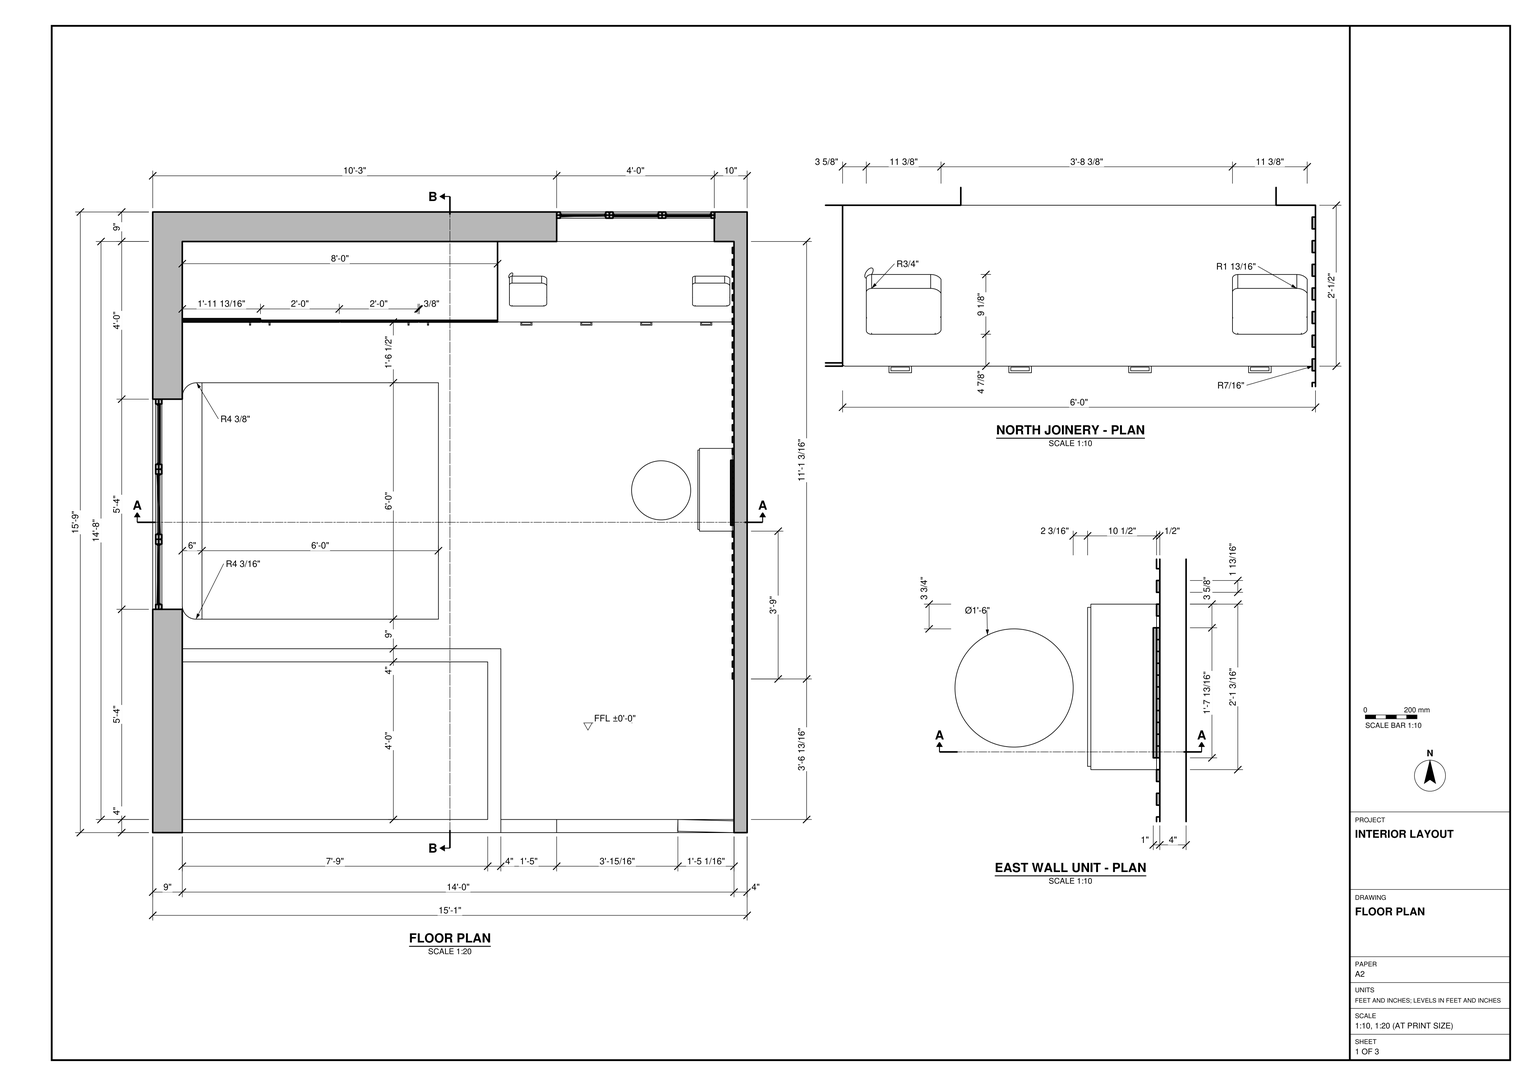
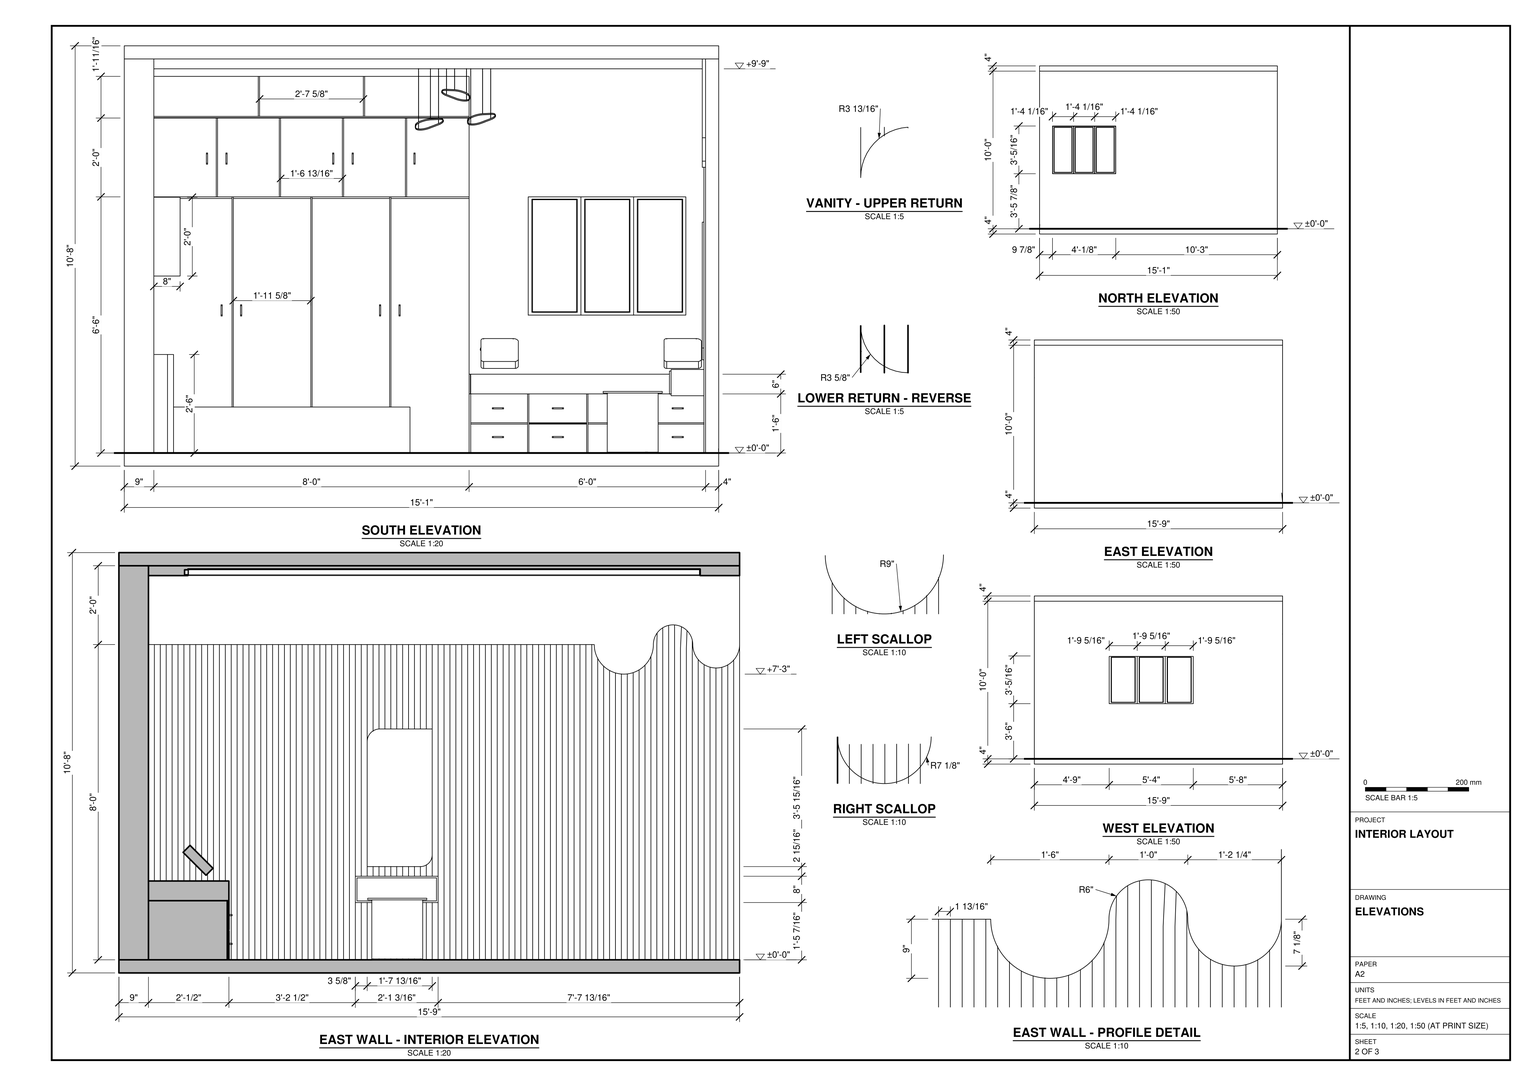
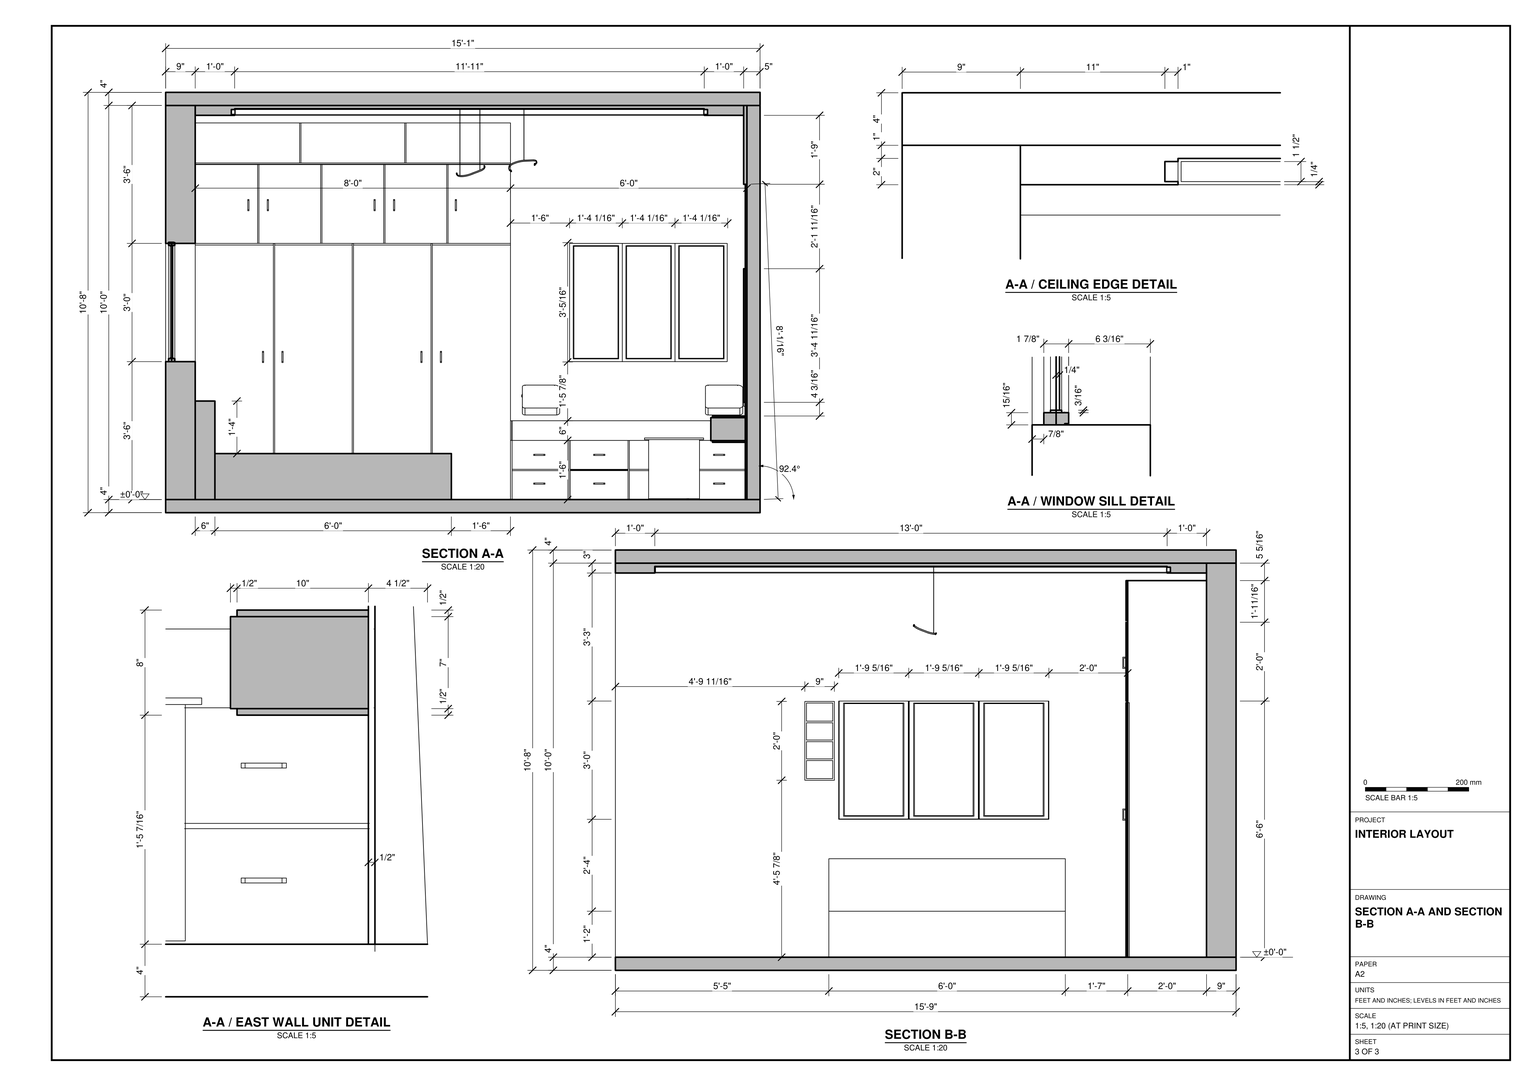
Build the bedroom interior in SketchUp from task_files/diagram_01.pdf. Work in feet and inches. Set the finished floor at ±0'-0". The overall model is 15'-1" east to west, 15'-9" north to south and 10'-8" high. Use the floor plan to locate the walls and furniture, and the elevations and sections to set their heights.

Model the floor slab, the 9" north and west walls, the 4" east wall and the top slab. Keep the south side open as drawn. Include the stepped ceiling edge and the three-panel window units in the north and west walls. Place the platform bed with its headboard against the west wall beneath the window. Along the north wall, fit the tall wardrobe and overhead cupboards beside the low drawer unit, keeping the opening below its counter in the position shown.

On the east wall, model the vertical ribs and follow the profile detail where their upper edge curves. Place the shallow dressing unit and mirror against this wall, with the round stool in front. Include the pendant lights in the position shown in elevation. Decor and loose items, including lights, may be any suitable library components.

Keep shell elements and each furniture or joinery piece in separate groups or components, and use components for repeated parts. Save one SketchUp model as output_files/bedroom_with_fitted_storage_and_a_dressing_area.skp.

# SketchUp Ruby script. Lengths in inches.
U = 1.inch
M = Sketchup.active_model
def pt(a) = Geom::Point3d.new(a.map { |v| v * U })
def face(e, loops, mat)
  f = e.add_face(loops[0].map { |a| pt(a) })
  loops[1..].each { |l| e.add_face(l.map { |a| pt(a) }).erase! }
  f.material = f.back_material = mat if mat
  f
end
# faces: each face lists its corners as indices into pts; further lists are holes
def faces(e, pts, list, mat = nil) = list.each { |f| face(e, (f[0].is_a?(Array) ? f : [f]).map { |l| l.map { |i| pts[i] } }, mat) }
# xy, xz, yz: faces in a plane at the given z, y or x. An outline is a flat list of corners, or four numbers for a rectangle; further outlines are holes
def ring(l) = l.size == 4 ? [[l[0], l[1]], [l[2], l[1]], [l[2], l[3]], [l[0], l[3]]] : l.each_slice(2).to_a
def flat(e, list, mat, &to3) = list.each { |f| face(e, (f[0].is_a?(Array) ? f : [f]).map { |l| ring(l).map { |u, v| to3.(u, v) } }, mat) }
def xy(e, z, list, mat = nil) = flat(e, list, mat) { |x, y| [x, y, z] }
def xz(e, y, list, mat = nil) = flat(e, list, mat) { |x, z| [x, y, z] }
def yz(e, x, list, mat = nil) = flat(e, list, mat) { |y, z| [x, y, z] }
def lines(e, pts, list) = list.each { |a, b| e.add_line(pt(pts[a]), pt(pts[b])) }
# prism: a flat outline (further loops are holes) pulled along v
def prism(e, loops, v, mat = nil)
  f = face(e, loops, mat); d = Geom::Vector3d.new(v.map { |x| x * U })
  f.pushpull(f.normal.samedirection?(d) ? d.length : -d.length)
end
def box(e, o, s, mat = nil) = prism(e, [[o, [o[0] + s[0], o[1], o[2]], [o[0] + s[0], o[1] + s[1], o[2]], [o[0], o[1] + s[1], o[2]]]], [0, 0, s[2]], mat)
def at(x, y, z, deg = 0) = Geom::Transformation.translation(pt([x, y, z])) * Geom::Transformation.rotation(ORIGIN, Z_AXIS, deg.degrees)
def axes(o, x, y, z) = Geom::Transformation.new([*x, 0, *y, 0, *z, 0, *pt(o).to_a, 1])
def part(name) = M.definitions.add(name)
# library, detail: a bought-in or finely detailed component or shape, given as its bounding box
def library(name, o, s) = part(name).tap { |d| box(d.entities, o, s) }
def detail(e, o, s) = box(e.add_group.entities, o, s)
def put(e, d, t, mat = nil) = e.add_instance(d, t).tap { |i| i.material = mat if mat }
def group(e, t, mat = nil) = e.add_group.tap { |g| g.transformation = t; g.material = mat if mat }.entities
root = M.entities
M.materials.add("0130_Gainsboro").color = [39, 45, 50]
M.materials.add("Emissive").color = [240, 235, 85]
M.materials.add("Wine2").color = [0, 0, 0]
M.materials["Wine2"].alpha = 0
M.materials.add("[0055_LightGoldenrodYellow]").color = [250, 250, 210]
M.materials.add("[0066_Honeydew]").color = [240, 255, 240]
M.materials.add("[0067_PaleGreen]").color = [223, 240, 176]
M.materials.add("[0134_DimGray]").color = [105, 105, 105]
M.materials.add("[Aluminum]").color = [179, 179, 179]
M.materials.add("[Carpet Berber Multi]").color = [151, 134, 122]
M.materials.add("[Carpet Berber Pattern Gray]").color = [165, 165, 165]
M.materials.add("[Carpet Pattern Leaf Squares Tan]").color = [181, 154, 125]
M.materials.add("[Carpet Pattern Squares Multi]").color = [138, 129, 101]
M.materials.add("[Mirror 02]").color = [229, 229, 229]
M.materials.add("[Translucent Glass Sky Reflection]").color = [126, 138, 183]
M.materials["[Translucent Glass Sky Reflection]"].alpha = 0.52
c1 = library("Rectangle Light",[-5.15,-5.15,-5.15],[10.3,10.3,5.15])
c2 = library("pendants",[20.82,-32.18,-15.09],[139.89,104.33,117.98])
c3 = part("Wardrobe door panel")
xy(c3.entities,0,[[0,-0.98,43.07,0],[0,0,43.07,1.4]],"0130_Gainsboro")
xy(c3.entities,0.3,[[0.3,-1.43,42.77,-0.98]],"0130_Gainsboro")
xy(c3.entities,2.95,[[2.95,-1.43,40.12,-0.63],[2.95,-0.63,40.12,0],[2.95,0,40.12,0.64],[2.95,0.64,40.12,1.4]],"0130_Gainsboro")
xy(c3.entities,3.54,[[3.54,-0.63,39.53,0],[3.54,0,39.53,0.64]],"0130_Gainsboro")
xy(c3.entities,111.8125,[[3.54,-0.63,39.53,0],[3.54,0,39.53,0.64]],"0130_Gainsboro")
xy(c3.entities,112.4,[[2.95,-1.43,40.12,-0.63],[2.95,-0.63,40.12,0],[2.95,0,40.12,0.64],[2.95,0.64,40.12,1.4]],"0130_Gainsboro")
xy(c3.entities,115.05,[[0.3,-1.43,42.77,-0.98]],"0130_Gainsboro")
xy(c3.entities,115.35,[[0,-0.98,43.07,0],[0,0,43.07,1.4]],"0130_Gainsboro")
xz(c3.entities,-1.43,[[[0.3,0.3,42.77,115.05],[2.95,2.95,40.12,112.4]]],"0130_Gainsboro")
xz(c3.entities,-0.98,[[[0,0,43.07,115.35],[0.3,0.3,42.77,115.05]]],"0130_Gainsboro")
xz(c3.entities,-0.63,[[[2.95,2.95,40.12,112.4],[3.54,3.54,39.53,111.8125]]],"0130_Gainsboro")
xz(c3.entities,0,[[[0,0,43.07,115.35],[2.95,2.95,40.12,112.4]],[[2.95,2.95,40.12,112.4],[3.54,3.54,39.53,111.8125]]],"0130_Gainsboro")
xz(c3.entities,0,[[3.54,3.54,39.53,111.8125]],"Wine2")
xz(c3.entities,0.64,[[[2.95,2.95,40.12,112.4],[3.54,3.54,39.53,111.8125]]],"0130_Gainsboro")
xz(c3.entities,1.4,[[[0,0,43.07,115.35],[2.95,2.95,40.12,112.4]]],"0130_Gainsboro")
yz(c3.entities,0,[[-0.98,0,0,115.35],[0,0,1.4,115.35]],"0130_Gainsboro")
yz(c3.entities,0.3,[[-1.43,0.3,-0.98,115.05]],"0130_Gainsboro")
yz(c3.entities,2.95,[[-1.43,2.95,-0.63,112.4],[-0.63,2.95,0,112.4],[0,2.95,0.64,112.4],[0.64,2.95,1.4,112.4]],"0130_Gainsboro")
yz(c3.entities,3.54,[[-0.63,3.54,0,111.8125],[0,3.54,0.64,111.8125]],"0130_Gainsboro")
yz(c3.entities,39.53,[[-0.63,3.54,0,111.8125],[0,3.54,0.64,111.8125]],"0130_Gainsboro")
yz(c3.entities,40.12,[[-1.43,2.95,-0.63,112.4],[-0.63,2.95,0,112.4],[0,2.95,0.64,112.4],[0.64,2.95,1.4,112.4]],"0130_Gainsboro")
yz(c3.entities,42.77,[[-1.43,0.3,-0.98,115.05]],"0130_Gainsboro")
yz(c3.entities,43.07,[[-0.98,0,0,115.35],[0,0,1.4,115.35]],"0130_Gainsboro")
c4 = part("Wardrobe door assembly")
put(c4.entities,c3,axes([90.57,1.43,0],[1.05148,0,0],[0,1,0],[0,0,1]))
put(c4.entities,c3,axes([0,1.43,0],[1.05148,0,0],[0,1,0],[0,0,1]))
put(c4.entities,c3,axes([45.29,1.43,0],[1.05148,0,0],[0,1,0],[0,0,1]))
c5 = part("Group\#8")
prism(c5.entities,[[[0,1,3.4375],[0,1,0],[0,0,0],[0,0,3.4375]],[[0,0.86,3.14],[0,0.29,3.14],[0,0.29,0.33],[0,0.86,0.33]]],[0.375,0,0])
c6 = library("Group\#13",[0,0,0],[1,180,33])
c7 = library("Group\#17",[0,0,0],[15.5,15.5,18])
c8 = library("Group\#18",[0,0,0],[18,18,0.5])
xy(root,4,[[123,0,159.92,0,159.92,0.41,159.83,0.41,159.92,4,123,4],[177,0,177.09,3.59,159.92,4,159.92,0.41],[159.83,0.41,159.92,0.41,159.92,4],[9,155.5,32.8,156.5],[33.2,155.5,56.8,156],
  [57.2,155.5,80.8,156]])
xy(root,81.5,[[9,155.5,32.8,156.5],[33.2,155.5,56.8,156],[57.2,155.5,80.8,156]])
xz(root,156,[[33.2,4,56.8,81.5],[57.2,4,80.8,81.5]])
xz(root,156.5,[[9,4,32.8,81.5]])
xz(root,187.62,[[140.37,47.02,153.78,81.125],[156.42,47.02,169.83,81.125]],"[Translucent Glass Sky Reflection]")
yz(root,2.25,[[112.42,47.12,130.25,81.22]],"[Translucent Glass Sky Reflection]")
yz(root,9,[[155.5,4,156.5,81.5]])
yz(root,32.8,[[155.5,4,156.5,81.5]])
yz(root,33.2,[[155.5,4,156,81.5]])
yz(root,56.8,[[155.5,4,156,81.5]])
yz(root,57.2,[[155.5,4,156,81.5]])
yz(root,80.8,[[155.5,4,156,81.5]])
# 1 loose lines left out
p = [[124.32,187.62,81.125],[124.32,187.62,47.02],[137.73,188.05,47.02],[137.73,188.05,81.125],[1.83,87.58,47.12],[1.83,87.58,81.22],
  [1.4,69.75,81.22],[1.4,69.75,47.12],[2.25,91.09,47.11],[1.4,108.91,47.11],[1.4,108.91,81.22],[2.25,91.09,81.22]]
faces(root,p,[[0,1,2,3],[4,5,6,7],[8,9,10,11]],"[Translucent Glass Sky Reflection]")
put(root,c1,axes([15.1,9.07,120.99],[0.8,0,0],[0,0.8,0],[0,0,0.8]))
put(root,c1,axes([15.1,76.48,120.99],[0.8,0,0],[0,0.8,0],[0,0,0.8]))
put(root,c1,axes([15.1,143.89,120.99],[0.8,0,0],[0,0.8,0],[0,0,0.8]))
put(root,c1,axes([169.6,76.48,120.99],[0.8,0,0],[0,0.8,0],[0,0,0.8]))
put(root,c1,axes([169.6,143.89,120.99],[0.8,0,0],[0,0.8,0],[0,0,0.8]))
put(root,c1,axes([169.6,9.07,120.99],[0.8,0,0],[0,0.8,0],[0,0,0.8]))
put(root,c1,axes([140.91,173.9,121],[0.8,0,0],[0,0.8,0],[0,0,0.8]))
put(root,c2,axes([84.45,87.32,104.48],[0.18,0,0],[0,0.18,0],[0,0,0.18]))
put(root,c4,axes([2.78,68,46],[0,0.47107,0],[-0.6678,0,0],[0,0,0.315]))
put(root,c4,axes([171.15,189,45.9],[-0.35441,0,0],[0,-0.6678,0],[0,0,0.315]))
g1 = group(root,at(9,156,4))
xy(g1,0,[[0,0,96,24]])
xy(g1,114.6875,[[0,0,96,24]])
xz(g1,0,[[0,0,23.8,78],[23.8,0,24.2,78],[24.2,0,47.8,78],[47.8,0,48.2,78],[48.2,0,71.8,78],
  [71.8,0,72.2,78],[72.2,0,96,78],[0,78,96,102.125],[0,102.125,96,114.6875]])
xz(g1,24,[[0,0,96,114.6875]])
yz(g1,0,[[0,0,24,114.6875]])
yz(g1,96,[[0,0,24,114.6875]])
g2 = group(root,at(9,155.5,4),"[0055_LightGoldenrodYellow]")
box(g2,[19.4,0,78],[18.8,0.5,24])
box(g2,[38.6,0,78],[18.8,0.5,24])
box(g2,[57.8,0,78],[18.8,0.5,24])
xy(g2,78,[[0,0,19,0.5]])
xy(g2,102,[[0,0,19,0.5]])
xz(g2,0,[[0,0,23.8,77.5],[24.2,0,47.8,77.5],[48.2,0,71.8,77.5],[72.2,0,96,77.5],[[0,78,19,102],[16,87.9375,16.375,91.375]],
  [77,78,96,102],[16,87.9375,16.375,91.375]])
xz(g2,0.5,[[0,78,19,102]])
yz(g2,0,[[0,78,0.5,102]])
yz(g2,19,[[0,78,0.5,102]])
put(root,c5,at(25,154.5,91.9375),"[Aluminum]")
put(root,c5,at(30.9375,154.5,91.9375),"[Aluminum]")
put(root,c5,at(63.4375,154.5,91.9375),"[Aluminum]")
put(root,c5,at(69.375,154.5,91.9375),"[Aluminum]")
put(root,c5,at(29.46,154.5,45.71),"[Aluminum]")
put(root,c5,at(35.39,154.5,45.71),"[Aluminum]")
put(root,c5,at(77.71,154.5,45.71),"[Aluminum]")
put(root,c5,at(83.64,154.5,45.71),"[Aluminum]")
put(root,c5,at(88.1875,154.5,91.9375))
g3 = group(root,at(9,65,4),"[Carpet Berber Pattern Gray]")
xy(g3,0,[[4.03,0,3.64,0.03,3.38,0.07,3.25,0.1,3.125,0.13,3,0.17,2.875,0.2,2.75,0.25,2.63,0.29,2.51,0.34,2.39,0.4,2.27,0.45,2.16,0.51,2.04,0.58,1.82,0.72,1.72,0.79,1.61,0.875,1.51,0.96,1.41,1.04,1.3125,1.13,1.22,1.22,1.13,1.3125,1.04,1.41,0.96,1.51,0.875,1.61,0.79,1.72,0.72,1.82,0.58,2.04,0.51,2.16,0.45,2.27,0.4,2.39,0.34,2.51,0.29,2.63,0.25,2.75,0.2,2.875,0.17,3,0.13,3.125,0.1,3.25,0.07,3.38,0.03,3.64,0,4.03,0,67.77,0.02,68.05,0.03,68.18,0.05,68.32,0.08,68.45,0.11,68.59,0.17,68.85,0.21,68.98,0.36,69.37,0.42,69.49,0.48,69.62,0.54,69.74,0.61,69.86,0.68,69.97,0.75,70.09,0.83,70.2,0.92,70.31,1,70.42,1.18,70.62,1.38,70.82,1.58,71,1.69,71.08,1.8,71.17,1.91,71.25,2.03,71.32,2.14,71.39,2.26,71.46,2.38,71.52,2.51,71.58,2.63,71.64,3.02,71.79,3.15,71.83,3.41,71.89,3.55,71.92,3.68,71.95,3.82,71.97,3.95,71.98,4.23,72,6,72,6,0],[6,0,78,72]])
xy(g3,14,[[6,0,78,72]])
xy(g3,30,[[4.03,0,6,0,6,72,4.23,72,3.95,71.98,3.82,71.97,3.68,71.95,3.55,71.92,3.41,71.89,3.15,71.83,3.02,71.79,2.63,71.64,2.51,71.58,2.38,71.52,2.26,71.46,2.14,71.39,2.03,71.32,1.91,71.25,1.8,71.17,1.69,71.08,1.58,71,1.38,70.82,1.18,70.62,1,70.42,0.92,70.31,0.83,70.2,0.75,70.09,0.68,69.97,0.61,69.86,0.54,69.74,0.48,69.62,0.42,69.49,0.36,69.37,0.21,68.98,0.17,68.85,0.11,68.59,0.08,68.45,0.05,68.32,0.03,68.18,0.02,68.05,0,67.77,0,4.03,0.03,3.64,0.07,3.38,0.1,3.25,0.13,3.125,0.17,3,0.2,2.875,0.25,2.75,0.29,2.63,0.34,2.51,0.4,2.39,0.45,2.27,0.51,2.16,0.58,2.04,0.72,1.82,0.79,1.72,0.875,1.61,0.96,1.51,1.04,1.41,1.13,1.3125,1.22,1.22,1.3125,1.13,1.41,1.04,1.51,0.96,1.61,0.875,1.72,0.79,1.82,0.72,2.04,0.58,2.16,0.51,2.27,0.45,2.39,0.4,2.51,0.34,2.63,0.29,2.75,0.25,2.875,0.2,3,0.17,3.125,0.13,3.25,0.1,3.38,0.07,3.64,0.03]])
xz(g3,0,[[4.03,0,4.16,30],[4.16,0,6,30],[6,0,78,14]])
xz(g3,72,[[4.23,0,4.37,30],[4.37,0,6,30],[6,0,78,14]])
yz(g3,0,[[4.03,0,4.16,30],[4.16,0,67.63,30],[67.63,0,67.77,30]])
yz(g3,6,[[0,0,72,14],[0,14,72,30]])
yz(g3,78,[[0,0,72,14]])
# 2 loose lines left out
p = [[3.51,0.05,0],[3.64,0.03,0],[3.64,0.03,30],[3.51,0.05,30],[3.77,0.02,0],[3.77,0.02,30],
  [3.9,0.01,0],[3.9,0.01,30],[4.03,0,0],[4.03,0,30],[3,0.17,0],[3.125,0.13,0],
  [3.125,0.13,30],[3,0.17,30],[3.25,0.1,0],[3.25,0.1,30],[3.38,0.07,0],[3.38,0.07,30],
  [2.63,0.29,0],[2.75,0.25,0],[2.75,0.25,30],[2.63,0.29,30],[2.875,0.2,0],[2.875,0.2,30],
  [2.39,0.4,0],[2.51,0.34,0],[2.51,0.34,30],[2.39,0.4,30],[2.27,0.45,0],[2.27,0.45,30],
  [2.04,0.58,0],[2.16,0.51,0],[2.16,0.51,30],[2.04,0.58,30],[1.82,0.72,0],[1.93,0.65,0],
  [1.93,0.65,30],[1.82,0.72,30],[1.72,0.79,0],[1.72,0.79,30],[1.61,0.875,0],[1.61,0.875,30],
  [1.51,0.96,0],[1.51,0.96,30],[1.3125,1.13,0],[1.41,1.04,0],[1.41,1.04,30],[1.3125,1.13,30],
  [1.22,1.22,0],[1.22,1.22,30],[1.13,1.3125,0],[1.13,1.3125,30],[1.04,1.41,0],[1.04,1.41,30],
  [0.96,1.51,0],[0.96,1.51,30],[0.875,1.61,0],[0.875,1.61,30],[0.79,1.72,0],[0.79,1.72,30],
  [0.72,1.82,0],[0.72,1.82,30],[0.65,1.93,0],[0.65,1.93,30],[0.58,2.04,0],[0.58,2.04,30],
  [0.51,2.16,0],[0.51,2.16,30],[0.45,2.27,0],[0.45,2.27,30],[0.4,2.39,0],[0.4,2.39,30],
  [0.34,2.51,0],[0.34,2.51,30],[0.29,2.63,0],[0.29,2.63,30],[0.25,2.75,0],[0.25,2.75,30],
  [0.2,2.875,0],[0.2,2.875,30],[0.17,3,0],[0.17,3,30],[0.13,3.125,0],[0.13,3.125,30],
  [0.1,3.25,0],[0.1,3.25,30],[0.07,3.38,0],[0.07,3.38,30],[0.05,3.51,0],[0.05,3.51,30],
  [0.03,3.64,0],[0.03,3.64,30],[0.02,3.77,0],[0.02,3.77,30],[0.01,3.9,0],[0.01,3.9,30],
  [0,4.03,0],[0,4.03,30],[0.01,67.91,0],[0,67.77,0],[0,67.77,30],[0.01,67.91,30],
  [0.02,68.05,0],[0.02,68.05,30],[0.03,68.18,0],[0.03,68.18,30],[0.05,68.32,0],[0.05,68.32,30],
  [0.08,68.45,0],[0.08,68.45,30],[0.11,68.59,0],[0.11,68.59,30],[0.14,68.72,0],[0.14,68.72,30],
  [0.17,68.85,0],[0.17,68.85,30],[0.21,68.98,0],[0.21,68.98,30],[0.26,69.11,0],[0.26,69.11,30],
  [0.31,69.24,0],[0.31,69.24,30],[0.36,69.37,0],[0.36,69.37,30],[0.42,69.49,0],[0.42,69.49,30],
  [0.48,69.62,0],[0.48,69.62,30],[0.54,69.74,0],[0.54,69.74,30],[0.61,69.86,0],[0.61,69.86,30],
  [0.68,69.97,0],[0.68,69.97,30],[0.75,70.09,0],[0.75,70.09,30],[0.83,70.2,0],[0.83,70.2,30],
  [0.92,70.31,0],[0.92,70.31,30],[1,70.42,0],[1,70.42,30],[1.09,70.52,0],[1.09,70.52,30],
  [1.18,70.62,0],[1.18,70.62,30],[1.28,70.72,0],[1.28,70.72,30],[1.38,70.82,0],[1.38,70.82,30],
  [1.48,70.91,0],[1.48,70.91,30],[1.58,71,0],[1.58,71,30],[1.69,71.08,0],[1.69,71.08,30],
  [1.8,71.17,0],[1.8,71.17,30],[1.91,71.25,0],[1.91,71.25,30],[2.03,71.32,0],[2.03,71.32,30],
  [2.14,71.39,0],[2.14,71.39,30],[2.26,71.46,0],[2.26,71.46,30],[2.38,71.52,0],[2.38,71.52,30],
  [2.51,71.58,0],[2.51,71.58,30],[2.63,71.64,0],[2.63,71.64,30],[2.76,71.69,0],[2.76,71.69,30],
  [2.89,71.74,0],[2.89,71.74,30],[3.02,71.79,0],[3.02,71.79,30],[3.15,71.83,0],[3.15,71.83,30],
  [3.28,71.86,0],[3.28,71.86,30],[3.41,71.89,0],[3.41,71.89,30],[3.55,71.92,0],[3.55,71.92,30],
  [3.68,71.95,0],[3.68,71.95,30],[3.82,71.97,0],[3.82,71.97,30],[3.95,71.98,0],[3.95,71.98,30],
  [4.09,71.99,0],[4.09,71.99,30],[4.23,72,0],[4.23,72,30]]
faces(g3,p,[[0,1,2,3],[1,4,5,2],[4,6,7,5],[6,8,9,7],[10,11,12,13],[11,14,15,12],[14,16,17,15],[16,0,3,17],
  [18,19,20,21],[19,22,23,20],[22,10,13,23],[24,25,26,27],[25,18,21,26],[28,24,27,29],[30,31,32,33],[31,28,29,32],
  [34,35,36,37],[35,30,33,36],[38,34,37,39],[40,38,39,41],[42,40,41,43],[44,45,46,47],[45,42,43,46],[48,44,47,49],
  [50,48,49,51],[52,50,51,53],[54,52,53,55],[56,54,55,57],[58,56,57,59],[60,58,59,61],[62,60,61,63],[64,62,63,65],
  [66,64,65,67],[68,66,67,69],[70,68,69,71],[72,70,71,73],[74,72,73,75],[76,74,75,77],[78,76,77,79],[80,78,79,81],
  [82,80,81,83],[84,82,83,85],[86,84,85,87],[88,86,87,89],[90,88,89,91],[92,90,91,93],[94,92,93,95],[96,94,95,97],
  [98,99,100,101],[102,98,101,103],[104,102,103,105],[106,104,105,107],[108,106,107,109],[110,108,109,111],[112,110,111,113],[114,112,113,115],
  [116,114,115,117],[118,116,117,119],[120,118,119,121],[122,120,121,123],[124,122,123,125],[126,124,125,127],[128,126,127,129],[130,128,129,131],
  [132,130,131,133],[134,132,133,135],[136,134,135,137],[138,136,137,139],[140,138,139,141],[142,140,141,143],[144,142,143,145],[146,144,145,147],
  [148,146,147,149],[150,148,149,151],[152,150,151,153],[154,152,153,155],[156,154,155,157],[158,156,157,159],[160,158,159,161],[162,160,161,163],
  [164,162,163,165],[166,164,165,167],[168,166,167,169],[170,168,169,171],[172,170,171,173],[174,172,173,175],[176,174,175,177],[178,176,177,179],
  [180,178,179,181],[182,180,181,183],[184,182,183,185],[186,184,185,187],[188,186,187,189],[190,188,189,191],[192,190,191,193],[194,192,193,195]])
g4 = group(root,at(81.2,155.5,4))
xy(g4,0,[[0,0,23.8,0.5],[23.8,0.5,95.8,24.5]])
xy(g4,18,[[23.8,0.5,95.8,24.5]])
xy(g4,77.5,[[0,0,23.8,0.5]])
xz(g4,0.5,[[0,0,23.8,77.4],[23.8,0,24.3,18],[24.3,0,41.6,18],[41.6,0,42,18],[42,0,59.6,18],
  [59.6,0,60,18],[60,0,77.6,18],[77.6,0,78,18],[78,0,95.8,18],[0,77.4,23.8,77.5]])
xz(g4,24.5,[[23.8,0,95.8,18]])
yz(g4,0,[[0,0,0.5,77.4],[0,77.4,0.5,77.5]])
yz(g4,23.8,[[0,0,0.5,77.4],[0.5,0,24.5,18],[0,77.4,0.5,77.5]])
yz(g4,95.8,[[0.5,0,24.5,18]])
put(root,c5,axes([115.5,154.5,17.42],[0,0,1],[0,1,0],[-1,0,0]),"[Aluminum]")
put(root,c5,axes([133.75,154.5,17.42],[0,0,1],[0,1,0],[-1,0,0]),"[Aluminum]")
g5 = group(root,at(152,154.5,17.42),"[Aluminum]")
prism(g5,[[[-3.4375,1,0],[0,1,0],[0,0,0],[-3.4375,0,0]],[[-3.14,0.86,0],[-3.14,0.29,0],[-0.33,0.29,0],[-0.33,0.86,0]]],[0,0,0.375])
put(root,c5,axes([170.25,154.5,17.42],[0,0,1],[0,1,0],[-1,0,0]),"[Aluminum]")
put(root,c5,axes([115.5,154.5,8.67],[0,0,1],[0,1,0],[-1,0,0]),"[Aluminum]")
put(root,c5,axes([133.75,154.5,8.67],[0,0,1],[0,1,0],[-1,0,0]),"[Aluminum]")
put(root,c5,axes([170.25,154.5,8.67],[0,0,1],[0,1,0],[-1,0,0]),"[Aluminum]")
put(root,c5,axes([152,154.5,8.67],[0,0,1],[0,1,0],[-1,0,0]),"[Aluminum]")
g6 = group(root,at(105.5,155.5,4),"[0055_LightGoldenrodYellow]")
xy(g6,0,[[0,0,17.3,0.5],[17.7,0,35.3,0.5],[35.7,0,53.3,0.5],[53.7,0,71.5,0.5]])
xy(g6,8.8,[[0,0,17.3,0.5],[17.7,0,35.3,0.5],[35.7,0,53.3,0.5],[53.7,0,71.5,0.5]])
xy(g6,9.2,[[0,0,17.3,0.5],[17.7,0,35.3,0.5],[35.7,0,53.3,0.5],[53.7,0,71.5,0.5]])
xy(g6,18,[[0,0,17.3,0.5],[17.7,0,35.3,0.5],[35.7,0,53.3,0.5],[53.7,0,71.5,0.5]])
xz(g6,0,[[0,0,17.3,8.8],[17.7,0,35.3,8.8],[35.7,0,53.3,8.8],[53.7,0,71.5,8.8],[0,9.2,17.3,18],
  [17.7,9.2,35.3,18],[35.7,9.2,53.3,18],[53.7,9.2,71.5,18]])
xz(g6,0.5,[[0,0,17.3,8.8],[17.7,0,35.3,8.8],[35.7,0,53.3,8.8],[53.7,0,71.5,8.8],[0,8.8,17.3,9.2],
  [17.7,8.8,35.3,9.2],[35.7,8.8,53.3,9.2],[53.7,8.8,71.5,9.2],[0,9.2,17.3,18],[17.7,9.2,35.3,18],
  [35.7,9.2,53.3,18],[53.7,9.2,71.5,18]])
yz(g6,0,[[0,0,0.5,8.8],[0,9.2,0.5,18]])
yz(g6,17.3,[[0,0,0.5,8.8],[0,9.2,0.5,18]])
yz(g6,17.7,[[0,0,0.5,8.8],[0,9.2,0.5,18]])
yz(g6,35.3,[[0,0,0.5,8.8],[0,9.2,0.5,18]])
yz(g6,35.7,[[0,0,0.5,8.8],[0,9.2,0.5,18]])
yz(g6,53.3,[[0,0,0.5,8.8],[0,9.2,0.5,18]])
yz(g6,53.7,[[0,0,0.5,8.8],[0,9.2,0.5,18]])
yz(g6,71.5,[[0,0,0.5,8.8],[0,9.2,0.5,18]])
g7 = group(root,at(105,155.5,22),"[Carpet Berber Pattern Gray]")
xy(g7,0,[[0.39,0,0.37,0.01,0.3,0.02,0.24,0.05,0.18,0.09,0.13,0.13,0.09,0.18,0.05,0.24,0.02,0.3,0.01,0.37,0,0.39,0,24.5,72,24.5,72,0.32,71.99,0.26,71.93,0.16,71.88,0.11,71.84,0.08,71.78,0.04,71.73,0.02,71.61,0],[0.39,0,0.4375,0,0.5,0],[72,0.32,72.01,0.38,72.01,0.44,72,0.5],[0,0.39,0,0.5,0,0.4375]])
xy(g7,6,[[0.39,0,71.61,0,71.73,0.02,71.78,0.04,71.84,0.08,71.88,0.11,71.93,0.16,71.99,0.26,72,0.32,72,24.5,0,24.5,0,0.39,0.01,0.37,0.02,0.3,0.05,0.24,0.09,0.18,0.13,0.13,0.18,0.09,0.24,0.05,0.3,0.02,0.37,0.01]])
xz(g7,0,[[0.39,0,0.5,6],[0.5,0,71.61,6]])
xz(g7,24.5,[[0,0,72,6]])
yz(g7,0,[[0.39,0,0.5,6],[0.5,0,24.5,6]])
yz(g7,72,[[0.32,0,0.5,6],[0.5,0,24.5,6]])
p = [[0.18,0.09,0],[0.24,0.05,0],[0.24,0.05,6],[0.18,0.09,6],[0.3,0.02,0],[0.3,0.02,6],
  [0.37,0.01,0],[0.37,0.01,6],[0.39,0,0],[0.39,0,6],[71.61,0,0],[71.67,0.01,0],
  [71.67,0.01,6],[71.61,0,6],[71.73,0.02,0],[71.78,0.04,0],[71.78,0.04,6],[71.73,0.02,6],
  [71.84,0.08,0],[71.84,0.08,6],[0.09,0.18,0],[0.13,0.13,0],[0.13,0.13,6],[0.09,0.18,6],
  [71.88,0.11,0],[71.88,0.11,6],[71.93,0.16,0],[71.93,0.16,6],[0.02,0.3,0],[0.05,0.24,0],
  [0.05,0.24,6],[0.02,0.3,6],[71.96,0.21,0],[71.96,0.21,6],[71.99,0.26,0],[71.99,0.26,6],
  [0.01,0.37,0],[0.01,0.37,6],[72,0.32,0],[72,0.32,6],[0,0.39,0],[0,0.39,6]]
faces(g7,p,[[0,1,2,3],[1,4,5,2],[4,6,7,5],[6,8,9,7],[10,11,12,13],[14,15,16,17],[11,14,17,12],[15,18,19,16],
  [20,21,22,23],[21,0,3,22],[18,24,25,19],[24,26,27,25],[28,29,30,31],[29,20,23,30],[26,32,33,27],[32,34,35,33],
  [36,28,31,37],[34,38,39,35],[40,36,37,41]])
g8 = group(root,at(108.375,170.78,35.75),"[Carpet Pattern Squares Multi]")
prism(g8,[[[10.72,-8.3,-6],[1.05,-8.3,-6],[0.94,-8.3,-6],[0.84,-8.28,-5.98],[0.74,-8.26,-5.96],[0.64,-8.22,-5.93],[0.56,-8.18,-5.89],[0.48,-8.13,-5.84],[0.41,-8.08,-5.78],[0.35,-8.02,-5.72],[0.3,-7.95,-5.65],[0.27,-7.88,-5.58],[0.25,-7.81,-5.51],[0.24,-7.73,-5.43],[0.24,-1.89,0.41],[0.25,-1.82,0.48],[0.27,-1.74,0.56],[0.3,-1.67,0.625],[0.35,-1.6,0.69],[0.41,-1.54,0.76],[0.48,-1.49,0.8125],[0.56,-1.4375,0.86],[0.64,-1.4,0.9],[0.74,-1.36,0.9375],[0.84,-1.34,0.96],[0.94,-1.32,0.97],[1.05,-1.32,0.98],[10.04,-1.32,0.98],[10.2,-1.32,0.97],[10.37,-1.34,0.96],[10.53,-1.37,0.93],[10.6875,-1.41,0.89],[10.84,-1.46,0.84],[10.98,-1.52,0.78],[11.12,-1.59,0.71],[11.24,-1.67,0.63],[11.36,-1.76,0.54],[11.46,-1.85,0.44],[11.54,-1.95,0.34],[11.62,-2.0625,0.24],[11.62,-7.67,-5.37],[11.59,-7.73,-5.43],[11.5625,-7.79,-5.49],[11.52,-7.85,-5.55],[11.48,-7.9,-5.6],[11.44,-7.95,-5.66],[11.38,-8,-5.71],[11.32,-8.05,-5.75],[11.26,-8.1,-5.8],[11.19,-8.14,-5.84],[11.12,-8.17,-5.875],[11.05,-8.21,-5.91],[10.97,-8.24,-5.94],[10.89,-8.26,-5.97],[10.81,-8.28,-5.99]]],[0,-2.12,2.12])
# 12 loose lines left out
g9 = group(root,at(164.125,170.78,35.75),"[Carpet Pattern Squares Multi]")
prism(g9,[[[10.72,-8.3,-6],[1.05,-8.3,-6],[0.94,-8.3,-6],[0.84,-8.28,-5.98],[0.74,-8.26,-5.96],[0.64,-8.22,-5.93],[0.56,-8.18,-5.89],[0.48,-8.13,-5.84],[0.41,-8.08,-5.78],[0.35,-8.02,-5.72],[0.3,-7.95,-5.65],[0.27,-7.88,-5.58],[0.25,-7.81,-5.51],[0.24,-7.73,-5.43],[0.24,-1.89,0.41],[0.25,-1.82,0.48],[0.27,-1.74,0.56],[0.3,-1.67,0.625],[0.35,-1.6,0.69],[0.41,-1.54,0.76],[0.48,-1.49,0.8125],[0.56,-1.4375,0.86],[0.64,-1.4,0.9],[0.74,-1.36,0.9375],[0.84,-1.34,0.96],[0.94,-1.32,0.97],[1.05,-1.32,0.98],[10.04,-1.32,0.98],[10.2,-1.32,0.97],[10.37,-1.34,0.96],[10.53,-1.37,0.93],[10.6875,-1.41,0.89],[10.84,-1.46,0.84],[10.98,-1.52,0.78],[11.12,-1.59,0.71],[11.24,-1.67,0.63],[11.36,-1.76,0.54],[11.46,-1.85,0.44],[11.54,-1.95,0.34],[11.62,-2.0625,0.24],[11.62,-7.67,-5.37],[11.59,-7.73,-5.43],[11.5625,-7.79,-5.49],[11.52,-7.85,-5.55],[11.48,-7.9,-5.6],[11.44,-7.95,-5.66],[11.38,-8,-5.71],[11.32,-8.05,-5.75],[11.26,-8.1,-5.8],[11.19,-8.14,-5.84],[11.12,-8.17,-5.875],[11.05,-8.21,-5.91],[10.97,-8.24,-5.94],[10.89,-8.26,-5.97],[10.81,-8.28,-5.99]]],[0,-2.12,2.12])
g10 = group(root,at(9,24,0))
box(g10,[-9,-24,0],[181,189,4])
put(root,c6,at(176,0,91),"[0067_PaleGreen]")
g11 = group(root,at(0,56,4),"[0066_Honeydew]")
xy(g11,42,[[0,12,9,76],[123,124,171,133]])
xy(g11,78,[[0,12,9,76],[123,124,171,133]])
xy(g11,120,[[0,-56,9,-56,9,124,177,124,177,-56,181,-56,181,133,0,133]])
xz(g11,-56,[[0,0,9,120],[177,0,181,120]])
xz(g11,12,[[0,42,9,78]])
xz(g11,76,[[0,42,9,78]])
xz(g11,124,[[[9,0,177,120],[123,42,171,78]]])
xz(g11,133,[[[0,0,181,120],[123,42,171,78]]])
yz(g11,0,[[[-56,0,133,120],[12,42,76,78]]])
yz(g11,9,[[[-56,0,124,120],[12,42,76,78]]])
yz(g11,123,[[124,42,133,78]])
yz(g11,171,[[124,42,133,78]])
yz(g11,177,[[-56,0,124,120]])
yz(g11,181,[[-56,0,133,120]])
g12 = group(root,at(0,0,2.85),"[0134_DimGray]")
xy(g12,1.15,[[0,0,9,56],[9,0,106,0,106,56,9,56,9,52,102,52,102,4,9,4],[106,0,177,4],[9,4,102,52],[176.5,46.8,177,48.6],
  [176.5,50.4,177,52],[176.5,52,177,52.2],[176.5,54,177,55.8],[176.5,57.6,177,59.4],[176.5,61.2,177,63],
  [176.5,64.8,177,66.6],[176.5,68.4,177,70.2],[176.5,72,177,73.8],[176.5,75.6,177,77.4],[176.5,79.2,177,81],
  [176.5,82.8,177,84.6],[176.5,86.4,177,88.2],[176.5,90,177,91.8],[176.5,93.6,177,95.4],[176.5,97.2,177,99],
  [176.5,100.8,177,102.6],[176.5,104.4,177,106.2],[176.5,108,177,109.8],[176.5,111.6,177,113.4],[176.5,115.2,177,117],
  [176.5,118.8,177,120.6],[176.5,122.4,177,124.2],[176.5,126,177,127.8],[176.5,129.6,177,131.4],[176.5,133.2,177,135],
  [176.5,136.8,177,138.6],[176.5,140.4,177,142.2],[176.5,144,177,145.8],[176.5,147.6,177,149.4],[176.5,151.2,177,153],
  [176.5,154.8,177,156.6],[176.5,158.4,177,160.2],[176.5,162,177,163.8],[176.5,165.6,177,167.4],[176.5,169.2,177,171],
  [176.5,172.8,177,174.6],[176.5,176.4,177,178.2]])
xy(g12,97.15,[[176.5,46.8,177,48.6],[176.5,50.4,177,52.2],[176.5,54,177,55.8],[176.5,57.6,177,59.4],[176.5,61.2,177,63],
  [176.5,64.8,177,66.6],[176.5,68.4,177,70.2],[176.5,72,177,73.8],[176.5,75.6,177,77.4],[176.5,79.2,177,81],
  [176.5,82.8,177,84.6],[176.5,86.4,177,88.2],[176.5,90,177,91.8],[176.5,93.6,177,95.4],[176.5,97.2,177,99],
  [176.5,100.8,177,102.6],[176.5,104.4,177,106.2],[176.5,108,177,109.8],[176.5,111.6,177,113.4],[176.5,115.2,177,117],
  [176.5,118.8,177,120.6],[176.5,122.4,177,124.2],[176.5,126,177,127.8],[176.5,129.6,177,131.4],[176.5,133.2,177,135],
  [176.5,136.8,177,138.6],[176.5,140.4,177,142.2],[176.5,144,177,145.8],[176.5,147.6,177,149.4],[176.5,151.2,177,153],
  [176.5,154.8,177,156.6],[176.5,158.4,177,160.2],[176.5,162,177,163.8],[176.5,165.6,177,167.4],[176.5,169.2,177,171],
  [176.5,172.8,177,174.6],[176.5,176.4,177,178.2]])
xz(g12,46.8,[[176.5,1.15,177,96.29],[176.5,96.29,177,97.15]])
xz(g12,48.6,[[176.5,1.15,177,96.3],[176.5,96.3,177,97.15]])
xz(g12,50.4,[[176.5,1.15,177,96.31],[176.5,96.31,177,97.15]])
xz(g12,52.2,[[176.5,1.15,177,96.33],[176.5,96.33,177,97.15]])
xz(g12,54,[[176.5,1.15,177,96.34],[176.5,96.34,177,97.15]])
xz(g12,55.8,[[176.5,1.15,177,96.35],[176.5,96.35,177,97.15]])
xz(g12,57.6,[[176.5,1.15,177,96.36],[176.5,96.36,177,97.15]])
xz(g12,59.4,[[176.5,1.15,177,96.375],[176.5,96.375,177,97.15]])
xz(g12,61.2,[[176.5,1.15,177,96.38],[176.5,96.38,177,97.15]])
xz(g12,63,[[176.5,1.15,177,96.4],[176.5,96.4,177,97.15]])
xz(g12,64.8,[[176.5,1.15,177,96.41],[176.5,96.41,177,97.15]])
xz(g12,66.6,[[176.5,1.15,177,96.42],[176.5,96.42,177,97.15]])
xz(g12,68.4,[[176.5,1.15,177,96.43],[176.5,96.43,177,97.15]])
xz(g12,70.2,[[176.5,1.15,177,96.44],[176.5,96.44,177,97.15]])
xz(g12,72,[[176.5,1.15,177,96.45],[176.5,96.45,177,97.15]])
xz(g12,73.8,[[176.5,1.15,177,96.47],[176.5,96.47,177,97.15]])
xz(g12,75.6,[[176.5,1.15,177,96.48],[176.5,96.48,177,97.15]])
xz(g12,77.4,[[176.5,1.15,177,96.49],[176.5,96.49,177,97.15]])
xz(g12,79.2,[[176.5,1.15,177,96.5],[176.5,96.5,177,97.15]])
xz(g12,81,[[176.5,1.15,177,96.51],[176.5,96.51,177,97.15]])
xz(g12,82.8,[[176.5,1.15,177,96.52],[176.5,96.52,177,97.15]])
xz(g12,84.6,[[176.5,1.15,177,96.54],[176.5,96.54,177,97.15]])
xz(g12,86.4,[[176.5,1.15,177,96.55],[176.5,96.55,177,97.15]])
xz(g12,88.2,[[176.5,1.15,177,96.56],[176.5,96.56,177,97.15]])
xz(g12,90,[[176.5,1.15,177,96.57],[176.5,96.57,177,97.15]])
xz(g12,91.8,[[176.5,1.15,177,96.58],[176.5,96.58,177,97.15]])
xz(g12,93.6,[[176.5,1.15,177,96.59],[176.5,96.59,177,97.15]])
xz(g12,95.4,[[176.5,1.15,177,96.61],[176.5,96.61,177,97.15]])
xz(g12,97.2,[[176.5,1.15,177,96.62],[176.5,96.62,177,97.15]])
xz(g12,99,[[176.5,1.15,177,96.63],[176.5,96.63,177,97.15]])
xz(g12,100.8,[[176.5,1.15,177,96.64],[176.5,96.64,177,97.15]])
xz(g12,102.6,[[176.5,1.15,177,96.65],[176.5,96.65,177,97.15]])
xz(g12,104.4,[[176.5,1.15,177,96.66],[176.5,96.66,177,97.15]])
xz(g12,106.2,[[176.5,1.15,177,96.68],[176.5,96.68,177,97.15]])
xz(g12,108,[[176.5,1.15,177,96.6875],[176.5,96.6875,177,97.15]])
xz(g12,109.8,[[176.5,1.15,177,96.7],[176.5,96.7,177,97.15]])
xz(g12,111.6,[[176.5,1.15,177,96.71],[176.5,96.71,177,97.15]])
xz(g12,113.4,[[176.5,1.15,177,96.72],[176.5,96.72,177,97.15]])
xz(g12,115.2,[[176.5,1.15,177,96.73],[176.5,96.73,177,97.15]])
xz(g12,117,[[176.5,1.15,177,96.75],[176.5,96.75,177,97.15]])
xz(g12,118.8,[[176.5,1.15,177,96.76],[176.5,96.76,177,97.15]])
xz(g12,120.6,[[176.5,1.15,177,96.77],[176.5,96.77,177,97.15]])
xz(g12,122.4,[[176.5,1.15,177,96.78],[176.5,96.78,177,97.15]])
xz(g12,124.2,[[176.5,1.15,177,96.79],[176.5,96.79,177,97.15]])
xz(g12,126,[[176.5,1.15,177,96.8],[176.5,96.8,177,97.15]])
xz(g12,127.8,[[176.5,1.15,177,96.82],[176.5,96.82,177,97.15]])
xz(g12,129.6,[[176.5,1.15,177,96.83],[176.5,96.83,177,97.15]])
xz(g12,131.4,[[176.5,1.15,177,96.84],[176.5,96.84,177,97.15]])
xz(g12,133.2,[[176.5,1.15,177,96.85],[176.5,96.85,177,97.15]])
xz(g12,135,[[176.5,1.15,177,96.86],[176.5,96.86,177,97.15]])
xz(g12,136.8,[[176.5,1.15,177,96.875],[176.5,96.875,177,97.15]])
xz(g12,138.6,[[176.5,1.15,177,96.89],[176.5,96.89,177,97.15]])
xz(g12,140.4,[[176.5,1.15,177,96.9],[176.5,96.9,177,97.15]])
xz(g12,142.2,[[176.5,1.15,177,96.91],[176.5,96.91,177,97.15]])
xz(g12,144,[[176.5,1.15,177,96.92],[176.5,96.92,177,97.15]])
xz(g12,145.8,[[176.5,1.15,177,96.93],[176.5,96.93,177,97.15]])
xz(g12,147.6,[[176.5,1.15,177,96.94],[176.5,96.94,177,97.15]])
xz(g12,149.4,[[176.5,1.15,177,96.96],[176.5,96.96,177,97.15]])
xz(g12,151.2,[[176.5,1.15,177,96.97],[176.5,96.97,177,97.15]])
xz(g12,153,[[176.5,1.15,177,96.98],[176.5,96.98,177,97.15]])
xz(g12,154.8,[[176.5,1.15,177,96.99],[176.5,96.99,177,97.15]])
xz(g12,156.6,[[176.5,1.15,177,97],[176.5,97,177,97.15]])
xz(g12,158.4,[[176.5,1.15,177,97.01],[176.5,97.01,177,97.15]])
xz(g12,160.2,[[176.5,1.15,177,97.03],[176.5,97.03,177,97.15]])
xz(g12,162,[[176.5,1.15,177,97.04],[176.5,97.04,177,97.15]])
xz(g12,163.8,[[176.5,1.15,177,97.05],[176.5,97.05,177,97.15]])
xz(g12,165.6,[[176.5,1.15,177,97.0625],[176.5,97.0625,177,97.15]])
xz(g12,167.4,[[176.5,1.15,177,97.07],[176.5,97.07,177,97.15]])
xz(g12,169.2,[[176.5,1.15,177,97.08],[176.5,97.08,177,97.15]])
xz(g12,171,[[176.5,1.15,177,97.1],[176.5,97.1,177,97.15]])
xz(g12,172.8,[[176.5,1.15,177,97.11],[176.5,97.11,177,97.15]])
xz(g12,174.6,[[176.5,1.15,177,97.12],[176.5,97.12,177,97.15]])
xz(g12,176.4,[[176.5,1.15,177,97.13],[176.5,97.13,177,97.15]])
xz(g12,178.2,[[176.5,1.15,177,97.14],[176.5,97.14,177,97.15]])
yz(g12,176.5,[[46.8,1.15,48.6,97.15],[50.4,1.15,52.2,97.15],[54,1.15,55.8,97.15],[57.6,1.15,59.4,97.15],[61.2,1.15,63,97.15],
  [64.8,1.15,66.6,97.15],[68.4,1.15,70.2,97.15],[72,1.15,73.8,97.15],[75.6,1.15,77.4,97.15],[79.2,1.15,81,97.15],
  [82.8,1.15,84.6,97.15],[86.4,1.15,88.2,97.15],[90,1.15,91.8,97.15],[93.6,1.15,95.4,97.15],[97.2,1.15,99,97.15],
  [100.8,1.15,102.6,97.15],[104.4,1.15,106.2,97.15],[108,1.15,109.8,97.15],[111.6,1.15,113.4,97.15],[115.2,1.15,117,97.15],
  [118.8,1.15,120.6,97.15],[122.4,1.15,124.2,97.15],[126,1.15,127.8,97.15],[129.6,1.15,131.4,97.15],[133.2,1.15,135,97.15],
  [136.8,1.15,138.6,97.15],[140.4,1.15,142.2,97.15],[144,1.15,145.8,97.15],[147.6,1.15,149.4,97.15],[151.2,1.15,153,97.15],
  [154.8,1.15,156.6,97.15],[158.4,1.15,160.2,97.15],[162,1.15,163.8,97.15],[165.6,1.15,167.4,97.15],[169.2,1.15,171,97.15],
  [172.8,1.15,174.6,97.15],[176.4,1.15,178.2,97.15]])
yz(g12,177,[[45,1.15,46.8,97.15],[48.6,1.15,50.4,97.15],[52.2,1.15,54,97.15],[55.8,1.15,57.6,97.15],[59.4,1.15,61.2,97.15],
  [63,1.15,64.8,97.15],[66.6,1.15,68.4,97.15],[70.2,1.15,72,97.15],[73.8,1.15,75.6,97.15],[77.4,1.15,79.2,97.15],
  [81,1.15,82.8,97.15],[84.6,1.15,86.4,97.15],[88.2,1.15,90,97.15],[91.8,1.15,93.6,97.15],[95.4,1.15,97.2,97.15],
  [99,1.15,100.8,97.15],[102.6,1.15,104.4,97.15],[106.2,1.15,108,97.15],[109.8,1.15,111.6,97.15],[113.4,1.15,115.2,97.15],
  [117,1.15,118.8,97.15],[120.6,1.15,122.4,97.15],[124.2,1.15,126,97.15],[127.8,1.15,129.6,97.15],[131.4,1.15,133.2,97.15],
  [135,1.15,136.8,97.15],[138.6,1.15,140.4,97.15],[142.2,1.15,144,97.15],[145.8,1.15,147.6,97.15],[149.4,1.15,151.2,97.15],
  [153,1.15,154.8,97.15],[156.6,1.15,158.4,97.15],[160.2,1.15,162,97.15],[163.8,1.15,165.6,97.15],[167.4,1.15,169.2,97.15],
  [171,1.15,172.8,97.15],[174.6,1.15,176.4,97.15],[178.2,1.15,180,97.15]])
# 159 loose lines left out
g13 = group(root,at(176,93.6,32.38),"[Mirror 02]")
prism(g13,[[[0.5,3.6,0],[0.5,19.8,0],[0.5,19.8,38.09],[0.5,19.77,38.57],[0.5,19.68,39.05],[0.5,19.53,39.5],[0.5,19.32,39.9375],[0.5,19.07,40.35],[0.5,18.76,40.72],[0.5,18.41,41.05],[0.5,18.02,41.33],[0.5,17.59,41.56],[0.5,17.15,41.74],[0.5,16.68,41.86],[0.5,16.2,41.91],[0.5,0,41.91],[0.5,0,3.6],[0.5,0.03,3.13],[0.5,0.12,2.67],[0.5,0.27,2.22],[0.5,0.48,1.8],[0.5,0.74,1.41],[0.5,1.05,1.05],[0.5,1.41,0.74],[0.5,1.8,0.48],[0.5,2.22,0.27],[0.5,2.67,0.12],[0.5,3.13,0.03]]],[-0.5,0,0])
g14 = group(root,at(166.5,91.8,21.4375),"[0055_LightGoldenrodYellow]")
xy(g14,0,[[0,0,10,25.2]])
xy(g14,0.5,[[-0.5,0.5,0,24.7],[0,0.5,10,24.7]])
xy(g14,7.5,[[-0.5,0.5,0,24.7],[0,0.5,10,24.7]])
xy(g14,8,[[0,0,10,25.2]])
xz(g14,0,[[0,0,10,8]])
xz(g14,0.5,[[-0.5,0.5,0,7.5],[0,0.5,10,7.5]])
xz(g14,24.7,[[-0.5,0.5,0,7.5],[0,0.5,10,7.5]])
xz(g14,25.2,[[0,0,10,8]])
yz(g14,-0.5,[[0.5,0.5,24.7,7.5]])
yz(g14,0,[[[0,0,25.2,8],[0.5,0.5,24.7,7.5]]])
yz(g14,10,[[[0,0,25.2,8],[0.5,0.5,24.7,7.5]]])
put(root,c7,at(147.0625,96.49,4.25),"[Carpet Berber Multi]")
put(root,c8,at(145.8125,95.24,22.25),"[Carpet Pattern Leaf Squares Tan]")
g15 = group(root,at(9,57.6875,57.89),"[0055_LightGoldenrodYellow]")
prism(g15,[[[0,9,0],[0,0,0],[0,0,24],[0,9,24]],[[0,8.5,0.5],[0,8.5,6],[0,0.5,6],[0,0.5,0.5]],[[0,0.5,23.5],[0,0.5,18],[0,8.5,18],[0,8.5,23.5]],[[0,8.5,6.5],[0,8.5,11.75],[0,0.5,11.75],[0,0.5,6.5]],[[0,8.5,12.25],[0,8.5,17.5],[0,0.5,17.5],[0,0.5,12.25]]],[8,0,0])
g16 = group(root,at(0,0,124))
box(g16,[0,0,0],[181,189,4])
g17 = group(root,at(9,155.5,82),"[0055_LightGoldenrodYellow]")
xy(g17,0,[[77,0,96,0.5]])
xy(g17,24.5,[[31.8,0,32.2,0.5],[63.8,0,64.2,0.5]])
xy(g17,36.6875,[[0,0,31.8,0.5],[32.2,0,63.8,0.5],[64.2,0,96,0.5]])
xz(g17,0,[[0,24.5,31.8,36.6875],[32.2,24.5,63.8,36.6875],[64.2,24.5,96,36.6875]])
xz(g17,0.5,[[77,0,77,24,0,24,0,36.6875,31.8,36.6875,31.8,24.5,32.2,24.5,32.2,36.6875,63.8,36.6875,63.8,24.5,64.2,24.5,64.2,36.6875,96,36.6875,96,0]])
yz(g17,31.8,[[0,24.5,0.5,36.6875]])
yz(g17,32.2,[[0,24.5,0.5,36.6875]])
yz(g17,63.8,[[0,24.5,0.5,36.6875]])
yz(g17,64.2,[[0,24.5,0.5,36.6875]])
yz(g17,77,[[0,0,0.5,24]])
yz(g17,96,[[0,0,0.5,24],[0,24.5,0.5,36.6875]])
# 2 loose lines left out
g18 = group(root,at(9,0,121))
xy(g18,0,[[[0,0,167,180],[12,12,155,168]]])
xy(g18,0.24,[[11,12.24,12,167.76],[155,12.24,156,167.76],[12.24,168,154.76,169]])
xy(g18,1.76,[[11,12.24,12,167.76],[155,12.24,156,167.76],[12.24,168,154.76,169]])
xy(g18,2,[[12,12,155,168]])
xy(g18,3,[[0,0,167,180]])
xz(g18,0,[[0,0,167,3]])
xz(g18,12,[[12,0,155,2]])
xz(g18,12.24,[[11,0.24,12,1.76],[155,0.24,156,1.76]])
xz(g18,167.76,[[11,0.24,12,1.76],[155,0.24,156,1.76]])
xz(g18,168,[[[12,0,155,2],[12.24,0.24,154.76,1.76]]])
xz(g18,169,[[12.24,0.24,154.76,1.76]],"Emissive")
xz(g18,180,[[0,0,167,3]])
yz(g18,0,[[0,0,180,3]])
yz(g18,11,[[12.24,0.24,167.76,1.76]],"Emissive")
yz(g18,12,[[[12,0,168,2],[12.24,0.24,167.76,1.76]]])
yz(g18,12.24,[[168,0.24,169,1.76]])
yz(g18,154.76,[[168,0.24,169,1.76]])
yz(g18,155,[[[12,0,168,2],[12.24,0.24,167.76,1.76]]])
yz(g18,156,[[12.24,0.24,167.76,1.76]],"Emissive")
yz(g18,167,[[0,0,180,3]])
